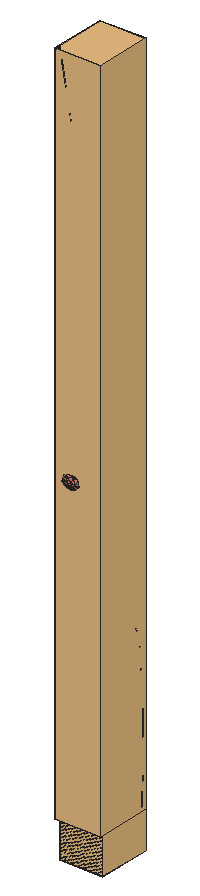
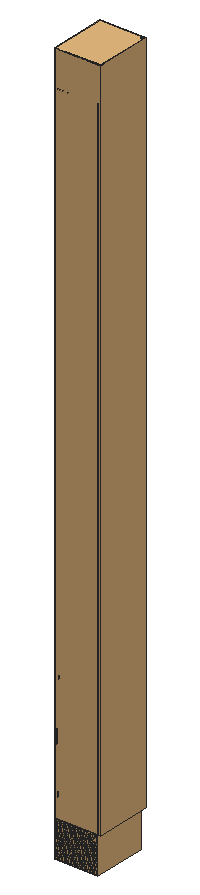
# SketchUp Ruby script. Lengths in inches.
U = 1.inch
M = Sketchup.active_model
def pt(a) = Geom::Point3d.new(a.map { |v| v * U })
def face(e, loops, mat)
  f = e.add_face(loops[0].map { |a| pt(a) })
  loops[1..].each { |l| e.add_face(l.map { |a| pt(a) }).erase! }
  f.material = f.back_material = mat if mat
  f
end
# faces: each face lists its corners as indices into pts; further lists are holes
def faces(e, pts, list, mat = nil) = list.each { |f| face(e, (f[0].is_a?(Array) ? f : [f]).map { |l| l.map { |i| pts[i] } }, mat) }
# xy, xz, yz: faces in a plane at the given z, y or x. An outline is a flat list of corners, or four numbers for a rectangle; further outlines are holes
def ring(l) = l.size == 4 ? [[l[0], l[1]], [l[2], l[1]], [l[2], l[3]], [l[0], l[3]]] : l.each_slice(2).to_a
def flat(e, list, mat, &to3) = list.each { |f| face(e, (f[0].is_a?(Array) ? f : [f]).map { |l| ring(l).map { |u, v| to3.(u, v) } }, mat) }
def xy(e, z, list, mat = nil) = flat(e, list, mat) { |x, y| [x, y, z] }
def xz(e, y, list, mat = nil) = flat(e, list, mat) { |x, z| [x, y, z] }
def yz(e, x, list, mat = nil) = flat(e, list, mat) { |y, z| [x, y, z] }
def lines(e, pts, list) = list.each { |a, b| e.add_line(pt(pts[a]), pt(pts[b])) }
# prism: a flat outline (further loops are holes) pulled along v
def prism(e, loops, v, mat = nil)
  f = face(e, loops, mat); d = Geom::Vector3d.new(v.map { |x| x * U })
  f.pushpull(f.normal.samedirection?(d) ? d.length : -d.length)
end
def box(e, o, s, mat = nil) = prism(e, [[o, [o[0] + s[0], o[1], o[2]], [o[0] + s[0], o[1] + s[1], o[2]], [o[0], o[1] + s[1], o[2]]]], [0, 0, s[2]], mat)
def at(x, y, z, deg = 0) = Geom::Transformation.translation(pt([x, y, z])) * Geom::Transformation.rotation(ORIGIN, Z_AXIS, deg.degrees)
def axes(o, x, y, z) = Geom::Transformation.new([*x, 0, *y, 0, *z, 0, *pt(o).to_a, 1])
def part(name) = M.definitions.add(name)
# library, detail: a bought-in or finely detailed component or shape, given as its bounding box
def library(name, o, s) = part(name).tap { |d| box(d.entities, o, s) }
def detail(e, o, s) = box(e.add_group.entities, o, s)
def put(e, d, t, mat = nil) = e.add_instance(d, t).tap { |i| i.material = mat if mat }
def group(e, t, mat = nil) = e.add_group.tap { |g| g.transformation = t; g.material = mat if mat }.entities
root = M.entities
M.materials.add("green").color = [174, 139, 102]
M.materials.add("vio").color = [206, 114, 100]
c1 = part("3DGeom~209_Defintion")
p = [[-82.63,99.78,-479.67],[16.24,-187.65,-448.99],[-197.0625,-62.73,-454.35],[148.38,0,-478.24],[-291.5,172.82,-352.58],[-2.625,262.29,-394.02],
  [-245.31,266.64,-303.125],[-291.5,172.82,-352.58],[-245.31,266.64,-303.125],[225.19,-262.29,-323.34],[339.63,-99.78,-348.66],[240.76,187.65,-379.34],
  [-120.25,-325.02,-299.44],[-315.27,-181.7,-324.83],[-120.25,-325.02,-299.44],[-357.57,78.99,-337.96],[-315.27,-181.7,-324.83],[-291.5,172.82,-352.58],
  [-357.57,78.99,-337.96],[106.99,-381.25,-193.82],[-120.25,-325.02,-299.44],[106.99,-381.25,-193.82],[21.51,381.25,-220.34],[-231.37,335.33,-202.85],
  [-2.625,262.29,-394.02],[-245.31,266.64,-303.125],[-231.37,335.33,-202.85],[21.51,381.25,-220.34],[-2.625,262.29,-394.02],[419.63,62.73,-263.01],
  [268.63,325.02,-178.79],[419.63,62.73,-263.01],[240.76,187.65,-379.34],[21.51,381.25,-220.34],[268.63,325.02,-178.79],[-291.5,172.82,-352.58],
  [-357.57,78.99,-337.96],[-422.26,199.55,-131.01],[-245.31,266.64,-303.125],[339.63,-99.78,-348.66],[373.81,-266.64,-111.04],[225.19,-262.29,-323.34],
  [339.63,-99.78,-348.66],[439.875,-172.82,-125.66],[373.81,-266.64,-111.04],[419.63,62.73,-263.01],[339.63,-99.78,-348.66],[-357.57,78.99,-337.96],
  [-315.27,-181.7,-324.83],[-425.81,10.31,-263.18],[-425.81,10.31,-263.18],[-315.27,-181.7,-324.83],[-224.52,-375.3,-69.66],[-405.57,-225.25,-125.83],
  [-315.27,-181.7,-324.83],[-120.25,-325.02,-299.44],[-315.27,-181.7,-324.83],[-405.57,-225.25,-125.83],[225.19,-262.29,-323.34],[305.5625,-335.33,-36.26],
  [106.99,-381.25,-193.82],[225.19,-262.29,-323.34],[373.81,-266.64,-111.04],[-231.37,335.33,-202.85],[16.69,-424.8,5.18],[-477.94,-14.83,-148.29],
  [419.63,62.73,-263.01],[486.07,-78.99,-76.21],[443.77,181.7,-89.33],[419.63,62.73,-263.01],[268.63,325.02,-178.79],[419.63,62.73,-263.01],
  [-16.69,424.8,-5.18],[268.63,325.02,-178.79],[-253.43,360.47,-78.63],[-231.37,335.33,-202.85],[-253.43,360.47,-78.63],[-253.43,360.47,-78.63],
  [253.43,-360.47,78.63],[224.52,375.3,69.66],[268.63,325.02,-178.79],[224.52,375.3,69.66],[268.63,325.02,-178.79],[-443.77,-181.7,89.33],
  [-500,10.31,-24.0625],[-486.07,78.99,76.21],[-439.875,172.82,125.66],[-373.81,266.64,111.04],[-305.5625,335.33,36.26],[-224.52,-375.3,-69.66],
  [-268.63,-325.02,178.79],[373.81,-266.64,-111.04],[422.26,-199.55,131.01],[305.5625,-335.33,-36.26],[373.81,-266.64,-111.04],[500,-10.31,24.0625],
  [405.57,225.25,125.83],[224.52,375.3,69.66],[-305.5625,335.33,36.26],[-253.43,360.47,-78.63],[-21.51,-381.25,220.34],[-21.51,-381.25,220.34],
  [-268.63,-325.02,178.79],[253.43,-360.47,78.63],[305.5625,-335.33,-36.26],[-419.63,-62.73,263.01],[-305.5625,335.33,36.26],[-106.99,381.25,193.82],
  [231.37,-335.33,202.85],[-21.51,-381.25,220.34],[477.94,14.83,148.29],[-373.81,266.64,111.04],[-305.5625,335.33,36.26],[120.25,325.02,299.44],
  [405.57,225.25,125.83],[-339.63,99.78,348.66],[231.37,-335.33,202.85],[253.43,-360.47,78.63],[-240.76,-187.65,379.34],[-240.76,-187.65,379.34],
  [-225.19,262.29,323.34],[-373.81,266.64,111.04],[-225.19,262.29,323.34],[-225.19,262.29,323.34],[315.27,181.7,324.83],[315.27,181.7,324.83],
  [405.57,225.25,125.83],[245.31,-266.64,303.125],[231.37,-335.33,202.85],[291.5,-172.82,352.58],[245.31,-266.64,303.125],[357.57,-78.99,337.96],
  [291.5,-172.82,352.58],[425.81,-10.31,263.18],[357.57,-78.99,337.96],[315.27,181.7,324.83],[-268.63,-325.02,178.79],[-21.51,-381.25,220.34],
  [2.625,-262.29,394.02],[-268.63,-325.02,178.79],[-240.76,-187.65,379.34],[-225.19,262.29,323.34],[120.25,325.02,299.44],[-106.99,381.25,193.82],
  [-21.51,-381.25,220.34],[245.31,-266.64,303.125],[-21.51,-381.25,220.34],[245.31,-266.64,303.125],[2.625,-262.29,394.02],[-419.63,-62.73,263.01],
  [-148.38,0,478.24],[-419.63,-62.73,263.01],[-339.63,99.78,348.66],[197.0625,62.74,454.35],[357.57,-78.99,337.96],[425.81,-10.31,263.18],
  [425.81,-10.31,263.18],[315.27,181.7,324.83],[-16.24,187.65,448.99],[315.27,181.7,324.83],[120.25,325.02,299.44],[-225.19,262.29,323.34],
  [120.25,325.02,299.44],[245.31,-266.64,303.125],[291.5,-172.82,352.58],[-339.63,99.78,348.66],[-225.19,262.29,323.34],[315.27,181.7,324.83],
  [82.63,-99.77,479.67],[-339.63,99.78,348.66]]
faces(c1.entities,p,[[0,1,2],[0,3,1],[4,0,2],[5,3,0],[6,0,7],[8,5,0],[3,9,1],[3,10,9],
  [11,10,3],[5,11,3],[2,12,13],[2,1,14],[15,2,16],[17,2,18],[1,19,20],[1,9,21],
  [22,11,5],[23,24,25],[26,27,28],[11,29,10],[30,31,32],[33,34,11],[35,36,37],[38,35,37],
  [39,40,41],[42,43,44],[45,43,46],[47,48,49],[36,50,37],[51,52,53],[54,55,52],[50,56,57],
  [58,59,60],[61,62,59],[63,38,37],[55,64,52],[55,60,64],[50,57,65],[50,65,37],[66,67,43],
  [68,67,69],[70,68,71],[72,73,27],[74,27,75],[76,72,27],[77,63,37],[60,78,64],[60,59,78],
  [79,68,80],[72,81,82],[65,57,83],[65,83,84],[65,84,37],[84,85,37],[85,86,37],[86,87,37],
  [88,77,37],[87,88,37],[57,89,90],[57,90,83],[91,43,92],[43,67,92],[93,94,92],[68,95,67],
  [96,95,68],[97,96,68],[98,72,99],[67,95,92],[52,64,100],[52,101,102],[103,104,92],[84,83,105],
  [84,105,85],[106,107,72],[107,81,72],[64,108,109],[64,78,108],[95,110,92],[96,110,95],[111,107,112],
  [113,114,81],[107,113,81],[85,105,115],[85,115,86],[116,117,92],[83,90,118],[83,119,105],[86,120,87],
  [121,122,107],[86,115,123],[124,110,96],[113,125,126],[127,128,92],[129,130,92],[131,132,92],[133,134,92],
  [110,133,92],[135,133,110],[136,137,138],[139,138,140],[141,142,143],[144,108,145],[146,147,148],[149,140,150],
  [151,150,152],[153,154,155],[153,156,157],[158,159,160],[161,158,162],[138,163,164],[165,158,166],[158,153,167],
  [168,164,154],[168,154,153],[169,150,158],[138,164,168],[140,138,168],[140,168,150],[150,153,158],[150,168,153]],"vio")
c2 = part("3DGeom~162_Defintion")
p = [[24.5,499.67,-28.18],[34.6875,499.96,-22.61],[27.51,499.8125,-29.5],[24.5,499.67,-28.18],[27.51,499.8125,-29.5],[25.94,499.74,-29.06],
  [27.51,499.8125,-29.5],[34.6875,499.96,-22.61],[30.68,499.93,-29.16],[27.51,499.8125,-29.5],[30.68,499.93,-29.16],[29.11,499.875,-29.54],
  [30.68,499.93,-29.16],[34.6875,499.96,-22.61],[33.33,499.99,-27.23],[30.68,499.93,-29.16],[33.33,499.99,-27.23],[32.11,499.97,-28.39],
  [22.58,499.54,-25.53],[34.6875,499.96,-22.61],[24.5,499.67,-28.18],[22.58,499.54,-25.53],[24.5,499.67,-28.18],[23.34,499.6,-26.96],
  [33.33,499.99,-27.23],[34.6875,499.96,-22.61],[34.66,499.99,-24.22],[33.33,499.99,-27.23],[34.66,499.99,-24.22],[34.21,500,-25.79],
  [22.24,499.47,-22.35],[34.6875,499.96,-22.61],[22.58,499.54,-25.53],[22.24,499.47,-22.35],[22.58,499.54,-25.53],[22.2,499.5,-23.96],
  [23.56,499.46,-19.35],[34.6875,499.96,-22.61],[22.24,499.47,-22.35],[26.22,499.53,-17.41],[34.6875,499.96,-22.61],[23.56,499.46,-19.35],
  [34.32,499.91,-21.05],[34.6875,499.96,-22.61],[26.22,499.53,-17.41],[23.56,499.46,-19.35],[22.24,499.47,-22.35],[22.6875,499.46,-20.79],
  [34.32,499.91,-21.05],[26.22,499.53,-17.41],[27.78,499.58,-17.04],[30.95,499.72,-17.52],[34.32,499.91,-21.05],[27.78,499.58,-17.04],
  [32.39,499.79,-18.39],[34.32,499.91,-21.05],[30.95,499.72,-17.52],[32.39,499.79,-18.39],[33.55,499.86,-19.61],[34.32,499.91,-21.05],
  [26.22,499.53,-17.41],[23.56,499.46,-19.35],[24.78,499.49,-18.1875],[30.95,499.72,-17.52],[27.78,499.58,-17.04],[29.39,499.65,-17.07],
  [-36.91,-499.89,26.6875],[-36.31,-499.93,26.63],[-35.71,-499.97,26.73],[-36.91,-499.89,26.6875],[-35.71,-499.97,26.73],[-34.01,-499.94,29.09],
  [-35.71,-499.97,26.73],[-35.15,-499.99,26.99],[-34.65,-500,27.39],[-35.71,-499.97,26.73],[-34.65,-500,27.39],[-34.01,-499.94,29.09],
  [-38,-499.78,27.26],[-37.49,-499.83,26.9],[-36.91,-499.89,26.6875],[-38,-499.78,27.26],[-36.91,-499.89,26.6875],[-34.01,-499.94,29.09],
  [-38.66,-499.67,28.32],[-38,-499.78,27.26],[-34.01,-499.94,29.09],[-38.66,-499.67,28.32],[-38.41,-499.72,27.75],[-38,-499.78,27.26],
  [-34.65,-500,27.39],[-34.29,-499.99,27.91],[-34.07,-499.97,28.49],[-34.65,-500,27.39],[-34.07,-499.97,28.49],[-34.01,-499.94,29.09],
  [-38.69,-499.59,29.52],[-38.66,-499.67,28.32],[-34.01,-499.94,29.09],[-38.69,-499.59,29.52],[-38.75,-499.625,28.91],[-38.66,-499.67,28.32],
  [-38.11,-499.57,30.62],[-38.69,-499.59,29.52],[-34.01,-499.94,29.09],[-37.06,-499.6,31.27],[-38.11,-499.57,30.62],[-34.01,-499.94,29.09],
  [-34.11,-499.9,29.69],[-37.06,-499.6,31.27],[-34.01,-499.94,29.09],[-38.11,-499.57,30.62],[-38.48,-499.57,30.1],[-38.69,-499.59,29.52],
  [-34.11,-499.9,29.69],[-36.46,-499.64,31.375],[-37.06,-499.6,31.27],[-35.28,-499.73,31.11],[-36.46,-499.64,31.375],[-34.11,-499.9,29.69],
  [-34.11,-499.9,29.69],[-34.76,-499.79,30.74],[-35.28,-499.73,31.11],[-34.11,-499.9,29.69],[-34.36,-499.85,30.25],[-34.76,-499.79,30.74],
  [-37.06,-499.6,31.27],[-37.62,-499.58,31.02],[-38.11,-499.57,30.62],[-35.28,-499.73,31.11],[-35.86,-499.68,31.32],[-36.46,-499.64,31.375]]
faces(c2.entities,p,[[0,1,2],[3,4,5],[6,7,8],[9,10,11],[12,13,14],[15,16,17],[18,19,20],[21,22,23],
  [24,25,26],[27,28,29],[30,31,32],[33,34,35],[36,37,38],[39,40,41],[42,43,44],[45,46,47],
  [48,49,50],[51,52,53],[54,55,56],[57,58,59],[60,61,62],[63,64,65],[66,67,68],[69,70,71],
  [72,73,74],[75,76,77],[78,79,80],[81,82,83],[84,85,86],[87,88,89],[90,91,92],[93,94,95],
  [96,97,98],[99,100,101],[102,103,104],[105,106,107],[108,109,110],[111,112,113],[114,115,116],[117,118,119],
  [120,121,122],[123,124,125],[126,127,128],[129,130,131]],"green")
c3 = library("3DGeom~76_Defintion",[-357.42,-500,-94.02],[714.84,1000,188.04])
c4 = part("3DGeom~77_Defintion")
p = [[339.625,495.99,-59.28],[344.32,486.75,-93.94],[336.28,491.02,-94.02],[339.625,495.99,-59.28],[336.28,491.02,-94.02],[329.77,495.38,-89.43],
  [339.625,495.99,-59.28],[351.73,483.72,-89.22],[344.32,486.75,-93.94],[339.625,495.99,-59.28],[329.77,495.38,-89.43],[326.53,498.67,-81.4],
  [339.625,495.99,-59.28],[356.52,482.74,-81.125],[351.73,483.72,-89.22],[339.625,495.99,-59.28],[326.53,498.67,-81.4],[327.42,500,-72.09],
  [339.625,495.99,-59.28],[357.42,484.07,-71.82],[356.52,482.74,-81.125],[339.625,495.99,-59.28],[327.42,500,-72.09],[332.22,499.02,-64],
  [339.625,495.99,-59.28],[354.18,487.36,-63.79],[357.42,484.07,-71.82],[339.625,495.99,-59.28],[347.66,491.72,-59.2],[354.18,487.36,-63.79],
  [-333.46,-489.29,27.51],[-350.37,-484.43,31.63],[-342.13,-486.03,27.33],[-323.61,-497.07,39.94],[-347.57,-495.14,60.61],[-333.46,-489.29,27.51],
  [-323.61,-497.07,39.94],[-333.46,-489.29,27.51],[-326.68,-493.33,32.125],[-333.46,-489.29,27.51],[-347.57,-495.14,60.61],[-350.37,-484.43,31.63],
  [-350.37,-484.43,31.63],[-347.57,-495.14,60.61],[-357.42,-487.36,48.18],[-350.37,-484.43,31.63],[-357.42,-487.36,48.18],[-355.96,-484.92,39.27],
  [-330.67,-500,56.48],[-347.57,-495.14,60.61],[-323.61,-497.07,39.94],[-330.67,-500,56.48],[-323.61,-497.07,39.94],[-325.07,-499.51,48.85],
  [-347.57,-495.14,60.61],[-354.35,-491.1,55.99],[-357.42,-487.36,48.18],[-347.57,-495.14,60.61],[-330.67,-500,56.48],[-338.9,-498.4,60.79]]
faces(c4.entities,p,[[0,1,2],[3,4,5],[6,7,8],[9,10,11],[12,13,14],[15,16,17],[18,19,20],[21,22,23],
  [24,25,26],[27,28,29],[30,31,32],[33,34,35],[36,37,38],[39,40,41],[42,43,44],[45,46,47],
  [48,49,50],[51,52,53],[54,55,56],[57,58,59]],"green")
c5 = library("3DGeom~161_Defintion",[-40.83,-526.88,-33.06],[81.66,1000,66.12])
c6 = library("3DGeom~158_Defintion",[-40.84,-526.87,-33.0625],[81.68,1000,66.125])
c7 = part("3DGeom~155_Defintion")
p = [[38.32,377.89,-31.94],[39.08,336.41,-30.625],[37.92,336.42,-31.72],[39.51,377.89,-30.8125],[36.28,473.1,-31.04],[39,423.46,-30.56],
  [37.77,423.45,-31.72],[36.57,299.05,-31.05],[35.37,265.71,-28.9],[34.28,265.75,-29.93],[37.7,299.02,-29.98],[37.54,473.12,-29.85],
  [30.51,238.44,-28.47],[26.13,217.53,-25.5625],[25.09,217.6875,-26.58],[31.58,238.34,-27.4375],[18.69,201.11,-24.24],[13.09,186.1875,-20.43],
  [12.09,186.36,-21.43],[19.71,200.92,-23.23],[17.34,-63.12,-14.97],[21.97,-83.66,-18.45],[21.09,-83.65,-19.17],[20.41,-107.24,-19.11],
  [17.68,-132.65,-15.82],[16.86,-132.61,-16.5],[21.25,-107.27,-18.41],[18.22,-63.09,-14.24],[5.95,170.98,-18.125],[1.85,152.3,-13.32],
  [0.82,152.32,-14.25],[6.97,170.87,-17.16],[11.42,-160.05,-12.18],[5.8,-189.86,-6.34],[5.02,-189.82,-6.98],[12.22,-160.09,-11.52],
  [-4.11,129.18,-8.57],[-8.33,104.16,-0.18],[-9.33,104.1,-1.06],[-3.09,129.2,-7.66],[0.27,-33.7,2.54],[10.55,-46.99,-6.22],
  [9.67,-47.04,-6.98],[1.16,-33.64,3.32],[-1.41,-222.19,-1.7],[-6.22,-257.42,3.45],[-6.96,-257.4,2.85],[-0.65,-222.22,-1.08],
  [-11.84,-295.59,6.88],[-16.11,-336.49,11.55],[-16.77,-336.48,11.01],[-11.14,-295.61,7.45],[-14.18,78.26,6.96],[-17,52.91,15.01],
  [-17.97,52.84,14.16],[-13.19,78.33,7.82],[-16.02,-7.84,18.13],[-7.97,-21.15,12.31],[-8.87,-21.22,11.51],[-15.1,-7.78,18.9375],
  [-21.76,-380.05,15.23],[-26.21,-426.32,20.02],[-26.8,-426.3,19.54],[-21.13,-380.0625,15.74],[-20.06,29.08,19.25],[-18.85,8.375,21.75],
  [-19.78,8.33,20.94],[-19.1,29.15,20.08],[-31.89,-475.25,23.94],[-36.52,-526.88,28.86],[-37.04,-526.87,28.4375],[-31.34,-475.26,24.4]]
faces(c7.entities,p,[[0,1,2],[0,3,1],[4,5,6],[7,8,9],[7,10,8],[4,11,5],[12,13,14],[12,15,13],
  [16,17,18],[16,19,17],[20,21,22],[23,24,25],[23,26,24],[20,27,21],[28,29,30],[28,31,29],
  [32,33,34],[32,35,33],[36,37,38],[36,39,37],[40,41,42],[40,43,41],[44,45,46],[44,47,45],
  [48,49,50],[48,51,49],[52,53,54],[52,55,53],[56,57,58],[56,59,57],[60,61,62],[60,63,61],
  [64,65,66],[64,67,65],[68,69,70],[68,71,69]],"green")
c8 = part("3DGeom~159_Defintion")
p = [[36.92,377.89,-32.7],[37.92,336.42,-31.72],[36.56,336.4375,-32.45],[38.32,377.89,-31.94],[34.8,473.07,-31.83],[37.77,423.44,-31.72],
  [36.34,423.43,-32.49],[35.25,299.08,-31.77],[34.28,265.75,-29.93],[32.99,265.81,-30.625],[36.57,299.05,-31.05],[36.28,473.1,-31.04],
  [39.51,377.89,-30.8125],[39.91,336.41,-29.26],[39.08,336.41,-30.625],[39.51,377.89,-30.8125],[40.37,377.89,-29.41],[37.53,473.12,-29.85],
  [39.87,423.46,-29.11],[39,423.45,-30.56],[37.7,299.02,-29.98],[36.15,265.7,-27.6],[35.37,265.71,-28.9],[37.7,299.02,-29.98],
  [38.51,299.02,-28.66],[37.53,473.12,-29.85],[38.43,473.12,-28.37],[29.25,238.59,-29.15],[25.09,217.6875,-26.58],[23.87,217.92,-27.27],
  [30.51,238.44,-28.47],[31.58,238.34,-27.4375],[26.875,217.45,-24.3],[26.13,217.52,-25.5625],[31.58,238.34,-27.4375],[32.35,238.29,-26.16],
  [17.52,201.39,-24.93],[12.09,186.36,-21.43],[10.92,186.63,-22.1],[18.69,201.11,-24.24],[19.71,200.92,-23.23],[13.83,186.13,-19.21],
  [13.09,186.1875,-20.43],[19.71,200.92,-23.23],[20.44,200.83,-21.98],[16.34,-63.24,-15.45],[21.09,-83.65,-19.17],[20.1,-83.67,-19.61],
  [19.4375,-107.2,-19.54],[16.86,-132.61,-16.5],[15.92,-132.54,-16.92],[20.41,-107.24,-19.11],[17.34,-63.12,-14.97],[4.77,171.17,-18.77],
  [0.82,152.32,-14.25],[-0.37,152.41,-14.87],[5.95,170.97,-18.125],[21.25,-107.27,-18.41],[18.3,-132.64,-14.94],[17.68,-132.65,-15.82],
  [21.25,-107.27,-18.41],[21.89,-107.28,-17.51],[18.22,-63.09,-14.24],[22.62,-83.68,-17.53],[21.97,-83.66,-18.45],[18.22,-63.09,-14.24],
  [18.89,-63.17,-13.31],[6.97,170.87,-17.16],[2.6,152.35,-12.15],[1.85,152.3,-13.32],[6.97,170.87,-17.16],[7.71,170.87,-15.96],
  [10.51,-159.96,-12.6],[5.02,-189.82,-6.98],[4.14,-189.74,-7.39],[11.42,-160.05,-12.18],[12.22,-160.09,-11.52],[6.39,-189.85,-5.52],
  [5.8,-189.86,-6.34],[12.22,-160.09,-11.52],[12.82,-160.08,-10.67],[-5.29,129.23,-9.17],[-9.33,104.1,-1.06],[-10.49,104.14,-1.64],
  [-4.11,129.17,-8.57],[-3.09,129.2,-7.66],[-7.59,104.3,0.93],[-8.33,104.16,-0.18],[-3.09,129.2,-7.66],[-2.34,129.3125,-6.53],
  [-0.69,-33.93,1.99],[9.67,-47.04,-6.98],[8.7,-47.23,-7.5],[0.27,-33.7,2.54],[1.16,-33.64,3.32],[11.25,-47.11,-5.29],
  [10.55,-46.99,-6.22],[1.16,-33.64,3.32],[1.875,-33.77,4.25],[-2.26,-222.12,-2.1],[-6.96,-257.4,2.85],[-7.79,-257.35,2.47],
  [-1.41,-222.19,-1.7],[-0.65,-222.22,-1.08],[-5.67,-257.41,4.22],[-6.22,-257.42,3.45],[-0.65,-222.22,-1.08],[-0.09,-222.21,-0.28],
  [-15.32,78.28,6.39],[-17.97,52.84,14.16],[-19.09,52.83,13.61],[-14.18,78.26,6.96],[-12.63,-295.55,6.52],[-16.77,-336.48,11.01],
  [-17.52,-336.4375,10.67],[-11.84,-295.59,6.88],[-11.14,-295.61,7.45],[-15.61,-336.49,12.25],[-16.11,-336.49,11.55],[-11.14,-295.61,7.45],
  [-10.62,-295.6,8.19],[-13.19,78.33,7.82],[-16.29,53.04,16.07],[-17,52.91,15.01],[-13.19,78.33,7.82],[-12.46,78.47,8.9],
  [-17.06,-8,17.6],[-8.87,-21.22,11.51],[-9.86,-21.4375,10.96],[-16.02,-7.84,18.13],[-15.1,-7.78,18.9375],[-7.26,-21.26,13.27],
  [-7.97,-21.15,12.31],[-15.1,-7.78,18.9375],[-14.41,-7.83,19.9375],[-22.47,-380.01,14.91],[-26.8,-426.3,19.54],[-27.47,-426.27,19.24],
  [-21.76,-380.05,15.23],[-21.13,-380.0625,15.74],[-25.76,-426.31,20.65],[-26.21,-426.32,20.02],[-21.13,-380.0625,15.74],[-20.66,-380.05,16.4],
  [-21.15,29.05,18.72],[-20.05,29.08,19.25],[-19.78,8.33,20.94],[-20.86,8.27,20.42],[-19.1,29.14,20.08],[-18.41,29.24,21.125],
  [-18.17,8.4,22.78],[-19.1,29.14,20.08],[-18.85,8.375,21.75],[-32.52,-475.22,23.66],[-37.04,-526.87,28.4375],[-37.63,-526.84,28.17],
  [-31.89,-475.24,23.94],[-31.33,-475.26,24.4],[-36.13,-526.875,29.41],[-36.52,-526.88,28.86],[-31.33,-475.26,24.4],[-30.92,-475.25,24.98]]
faces(c8.entities,p,[[0,1,2],[0,3,1],[4,5,6],[7,8,9],[7,10,8],[4,11,5],[12,13,14],[15,16,13],
  [17,18,19],[20,21,22],[23,24,21],[25,26,18],[27,28,29],[27,30,28],[31,32,33],[34,35,32],
  [36,37,38],[36,39,37],[40,41,42],[43,44,41],[45,46,47],[48,49,50],[48,51,49],[45,52,46],
  [53,54,55],[53,56,54],[57,58,59],[60,61,58],[62,63,64],[65,66,63],[67,68,69],[70,71,68],
  [72,73,74],[72,75,73],[76,77,78],[79,80,77],[81,82,83],[81,84,82],[85,86,87],[88,89,86],
  [90,91,92],[90,93,91],[94,95,96],[97,98,95],[99,100,101],[99,102,100],[103,104,105],[106,107,104],
  [108,109,110],[108,111,109],[112,113,114],[112,115,113],[116,117,118],[119,120,117],[121,122,123],[124,125,122],
  [126,127,128],[126,129,127],[130,131,132],[133,134,131],[135,136,137],[135,138,136],[139,140,141],[142,143,140],
  [144,145,146],[144,146,147],[148,149,150],[151,150,152],[153,154,155],[153,156,154],[157,158,159],[160,161,158]],"green")
c9 = part("3DGeom~240_Defintion")
p = [[-78.2,0,-500],[136.57,-186.02,-435.25],[-104.59,-107.4,-478.72],[182.28,0,-472.11],[-317.72,0,-393.91],[-104.59,107.4,-478.72],
  [11.71,-322.2,-334.53],[-176.68,-186.02,-420.57],[-176.68,186.02,-420.57],[136.57,186.02,-435.25],[341.14,-214.8,-275.16],[393.91,0,-317.72],
  [196.96,-372.05,-158.86],[196.96,-372.05,-158.86],[341.14,214.8,-275.16],[11.71,322.2,-334.54],[-158.86,-372.05,-196.96],[-275.16,-214.8,-341.14],
  [-275.16,214.8,-341.14],[-373.63,-186.02,-261.71],[-373.63,-186.02,-261.71],[-445.73,-107.4,-203.5625],[-317.72,0,-393.91],[-472.11,0,-182.28],
  [-317.72,0,-393.91],[-445.73,107.4,-203.5625],[-317.72,0,-393.91],[-373.63,186.02,-261.71],[-317.72,0,-393.91],[-373.63,186.02,-261.71],
  [-275.16,-214.8,-341.14],[-158.86,-372.05,-196.96],[-329.43,-322.2,-59.38],[-275.16,-214.8,-341.14],[-329.43,-322.2,-59.38],[-373.63,-186.02,-261.71],
  [-373.63,186.02,-261.71],[-158.86,372.04,-196.96],[-275.16,214.8,-341.14],[-158.86,372.04,-196.96],[11.71,-322.2,-334.53],[0,-429.6,0],
  [-158.86,-372.05,-196.96],[11.71,-322.2,-334.53],[196.96,-372.05,-158.86],[196.96,372.04,-158.86],[-158.86,372.04,-196.96],[196.96,372.04,-158.86],
  [11.71,322.2,-334.54],[393.91,0,-317.72],[454.3,-186.02,-41.34],[341.14,-214.8,-275.16],[393.91,0,-317.72],[500,0,-78.2],
  [341.14,214.8,-275.16],[393.91,0,-317.72],[341.14,-214.8,-275.16],[329.43,-322.2,59.38],[196.96,-372.05,-158.86],[341.14,-214.8,-275.16],
  [329.43,-322.2,59.38],[341.14,214.8,-275.16],[454.3,186.02,-41.34],[196.96,372.04,-158.86],[341.14,214.8,-275.16],[-329.43,-322.2,-59.38],
  [-454.3,-186.02,41.34],[-329.43,322.2,-59.38],[-373.63,186.02,-261.71],[-373.63,186.02,-261.71],[-329.43,322.2,-59.38],[-158.86,372.04,-196.96],
  [-500,0,78.2],[-454.3,186.02,41.34],[-329.43,322.2,-59.38],[-158.86,-372.05,-196.96],[-196.96,-372.04,158.86],[-158.86,-372.05,-196.96],
  [-196.96,-372.04,158.86],[-329.43,-322.2,-59.38],[0,429.6,0],[-158.86,372.04,-196.96],[-158.86,372.04,-196.96],[196.96,372.04,-158.86],
  [158.86,-372.04,196.96],[329.43,-322.2,59.38],[196.96,372.04,-158.86],[329.43,322.2,59.38],[329.43,322.2,59.38],[196.96,372.04,-158.86],
  [445.73,-107.4,203.5625],[472.11,0,182.28],[-196.96,-372.04,158.86],[-341.14,-214.8,275.16],[-196.96,372.05,158.86],[-329.43,322.2,-59.38],
  [-196.96,372.05,158.86],[373.63,-186.02,261.71],[329.43,-322.2,59.38],[373.63,-186.02,261.71],[445.73,107.4,203.5625],[-11.71,-322.2,334.54],
  [-196.96,-372.04,158.86],[-11.71,-322.2,334.54],[158.86,372.05,196.96],[329.43,322.2,59.38],[-393.91,0,317.72],[-341.14,214.8,275.16],
  [-196.96,372.05,158.86],[275.16,-214.8,341.14],[373.63,-186.02,261.71],[373.63,186.02,261.71],[373.63,186.02,261.71],[329.43,322.2,59.38],
  [-196.96,-372.04,158.86],[-136.57,-186.02,435.25],[-341.14,-214.8,275.16],[-196.96,-372.04,158.86],[-11.71,-322.2,334.54],[-341.14,214.8,275.16],
  [-11.71,322.2,334.53],[-196.96,372.05,158.86],[-11.71,322.2,334.53],[317.72,0,393.91],[317.72,0,393.91],[158.86,-372.04,196.96],
  [176.68,-186.02,420.57],[158.86,-372.04,196.96],[275.16,-214.8,341.14],[275.16,214.8,341.14],[373.63,186.02,261.71],[-11.71,322.2,334.53],
  [275.16,214.8,341.14],[158.86,372.05,196.96],[373.63,-186.02,261.71],[317.72,0,393.91],[317.72,0,393.91],[275.16,-214.8,341.14],
  [373.63,-186.02,261.71],[317.72,0,393.91],[373.63,186.02,261.71],[275.16,214.8,341.14],[-341.14,-214.8,275.16],[-182.28,0,472.11],
  [-393.91,0,317.72],[-341.14,-214.8,275.16],[-393.91,0,317.72],[-136.57,186.02,435.25],[-341.14,214.8,275.16],[-341.14,214.8,275.16],
  [-11.71,322.2,334.53],[-393.91,0,317.72],[104.59,-107.4,478.72],[176.68,186.02,420.57],[-11.71,322.2,334.53],[-11.71,322.2,334.53],
  [275.16,214.8,341.14],[275.16,-214.8,341.14],[275.16,214.8,341.14],[78.2,0,500],[104.59,107.4,478.72]]
faces(c9.entities,p,[[0,1,2],[0,3,1],[0,2,4],[5,0,4],[5,3,0],[2,6,7],[2,1,6],[2,7,4],
  [8,5,4],[5,9,3],[8,9,5],[3,10,1],[3,11,10],[9,11,3],[1,12,6],[1,10,13],
  [9,14,11],[8,15,9],[15,14,9],[7,16,17],[7,6,16],[7,17,4],[18,8,4],[18,15,8],
  [17,19,4],[20,21,22],[21,23,24],[23,25,26],[25,27,28],[29,18,4],[30,31,32],[33,34,35],
  [36,37,38],[18,39,15],[40,41,42],[43,44,41],[15,45,14],[46,47,48],[49,50,51],[52,53,50],
  [54,53,55],[56,57,58],[59,50,60],[61,62,53],[63,62,64],[20,65,66],[20,66,21],[25,67,68],
  [69,70,71],[21,66,72],[21,72,23],[23,73,25],[25,73,74],[75,41,76],[77,78,79],[70,80,81],
  [82,80,83],[23,72,73],[44,84,41],[44,85,84],[86,87,62],[80,88,89],[53,90,50],[53,91,90],
  [62,91,53],[65,92,93],[65,93,66],[73,94,95],[70,96,80],[50,97,98],[50,90,99],[62,100,91],
  [87,100,62],[41,101,102],[41,84,103],[80,104,105],[96,104,80],[66,93,106],[66,106,72],[72,107,73],
  [73,107,108],[85,109,84],[85,110,109],[87,111,100],[104,112,113],[72,106,107],[114,115,116],[117,118,115],
  [119,120,121],[96,122,104],[90,91,123],[91,100,124],[125,126,118],[127,128,126],[104,129,130],[131,132,133],
  [134,90,135],[100,111,136],[137,138,139],[140,141,139],[142,143,144],[145,115,143],[146,147,148],[149,147,150],
  [151,143,147],[118,152,115],[118,126,152],[147,153,154],[155,153,156],[126,157,139],[158,153,139],[152,126,139],
  [159,152,139],[160,159,139],[153,160,139],[147,160,153],[115,159,143],[115,152,159],[143,160,147],[143,159,160]],"vio")
c10 = library("3DGeom~160_Defintion",[-35.87,-474.24,-32.99],[76.62,1000,62.39])
c11 = library("3DGeom~156_Defintion",[-35.87,-474.23,-32.99],[76.62,1000,62.39])
c12 = part("3DGeom~154_Defintion")
p = [[37.69,422.55,-31.65],[39.43,377.09,-30.75],[38.24,377.08,-31.875],[37.84,335.71,-31.66],[37.62,298.39,-29.92],[36.5,298.41,-30.99],
  [39,335.7,-30.56],[38.91,422.56,-30.49],[33.77,525.73,-29.85],[37.46,472.11,-29.79],[36.2,472.09,-30.97],[34.2,265.19,-29.87],
  [31.51,237.83,-27.38],[30.44,237.9375,-28.41],[35.3,265.15,-28.83],[35.05,525.75,-28.63],[25.03,217.23,-26.53],[19.66,200.49,-23.18],
  [18.65,200.68,-24.19],[26.07,217.0625,-25.51],[12.06,185.97,-21.38],[6.95,170.51,-17.12],[5.93,170.61,-18.08],[13.07,185.79,-20.39],
  [21.05,-83.47,-19.125],[21.21,-107.04,-18.37],[20.36,-107.02,-19.07],[21.92,-83.48,-18.41],[16.82,-132.33,-16.46],[12.19,-159.75,-11.49],
  [11.4,-159.71,-12.15],[17.65,-132.37,-15.78],[9.65,-46.9375,-6.96],[18.18,-62.96,-14.21],[17.3,-62.98,-14.9375],[10.53,-46.89,-6.21],
  [0.82,152,-14.22],[-3.09,128.93,-7.65],[-4.1,128.9,-8.55],[1.84,151.98,-13.29],[5.01,-189.42,-6.97],[-0.65,-221.75,-1.08],
  [-1.4,-221.72,-1.7],[5.79,-189.46,-6.32],[-9.3125,103.88,-1.06],[-13.16,78.16,7.8],[-14.15,78.09,6.94],[-8.3125,103.94,-0.18],
  [-8.85,-21.17,11.49],[1.16,-33.57,3.31],[0.27,-33.63,2.53],[-6.94,-256.85,2.84],[-11.11,-294.98,7.4375],[-11.81,-294.96,6.87],
  [-6.21,-256.87,3.44],[-7.96,-21.11,12.28],[-16.73,-335.76,10.98],[-21.09,-379.25,15.71],[-21.71,-379.24,15.19],[-16.07,-335.78,11.53],
  [-17.94,52.72,14.13],[-19.0625,29.08,20.03],[-20.01,29.02,19.21],[-16.97,52.79,14.98],[-19.74,8.3125,20.9],[-15.07,-7.76,18.9],
  [-15.98,-7.82,18.1],[-18.8125,8.36,21.71],[-26.74,-425.4,19.5],[-31.27,-474.25,24.35],[-31.82,-474.23,23.89],[-26.15,-425.41,19.98]]
faces(c12.entities,p,[[0,1,2],[3,4,5],[3,6,4],[0,7,1],[8,9,10],[11,12,13],[11,14,12],[8,15,9],
  [16,17,18],[16,19,17],[20,21,22],[20,23,21],[24,25,26],[24,27,25],[28,29,30],[28,31,29],
  [32,33,34],[32,35,33],[36,37,38],[36,39,37],[40,41,42],[40,43,41],[44,45,46],[44,47,45],
  [48,49,50],[51,52,53],[51,54,52],[48,55,49],[56,57,58],[56,59,57],[60,61,62],[60,63,61],
  [64,65,66],[64,67,65],[68,69,70],[68,71,69]],"green")
g1 = group(root,at(15.3125,38.42,26.21))
put(g1,c1,axes([-1.13,-0.59,9.41],[0,0.00039,0],[0,0,-0.00039],[-0.00039,0,0]),"vio")
put(root,c2,axes([14.3,38.14,35.93],[0,0.01161,0],[0,0,-0.01161],[-0.01161,0,0]),"green")
g2 = group(root,at(15.3125,38.42,26.21))
put(g2,c3,axes([-1.1,-0.3,8.98],[0,0.00081,0],[0,0,-0.00081],[-0.00081,0,0]),"green")
put(g2,c4,axes([-1.1,-0.3,8.98],[0,0.00081,0],[0,0,-0.00081],[-0.00081,0,0]),"green")
put(root,c5,axes([14.3,38.14,35.93],[0,0.01102,0],[0,0,-0.01102],[-0.01102,0,0]),"green")
put(root,c6,axes([14.3,38.14,35.93],[0,0.01102,0],[0,0,-0.01102],[-0.01102,0,0]),"green")
put(root,c7,axes([14.3,38.14,35.93],[0,0.01102,0],[0,0,-0.01102],[-0.01102,0,0]),"green")
put(root,c8,axes([14.3,38.14,35.93],[0,0.01102,0],[0,0,-0.01102],[-0.01102,0,0]),"green")
g3 = group(root,at(15.3125,38.42,26.21))
put(g3,c9,axes([-0.96,-0.26,8.41],[0,0.00039,0],[0,0,-0.00039],[-0.00039,0,0]),"vio")
put(root,c10,axes([14.3,38.14,35.93],[0,0.01104,0],[0,0,-0.01104],[-0.01104,0,0]),"green")
put(root,c11,axes([14.3,38.14,35.93],[0,0.01104,0],[0,0,-0.01104],[-0.01104,0,0]),"green")
put(root,c12,axes([14.3,38.14,35.93],[0,0.01104,0],[0,0,-0.01104],[-0.01104,0,0]),"green")
